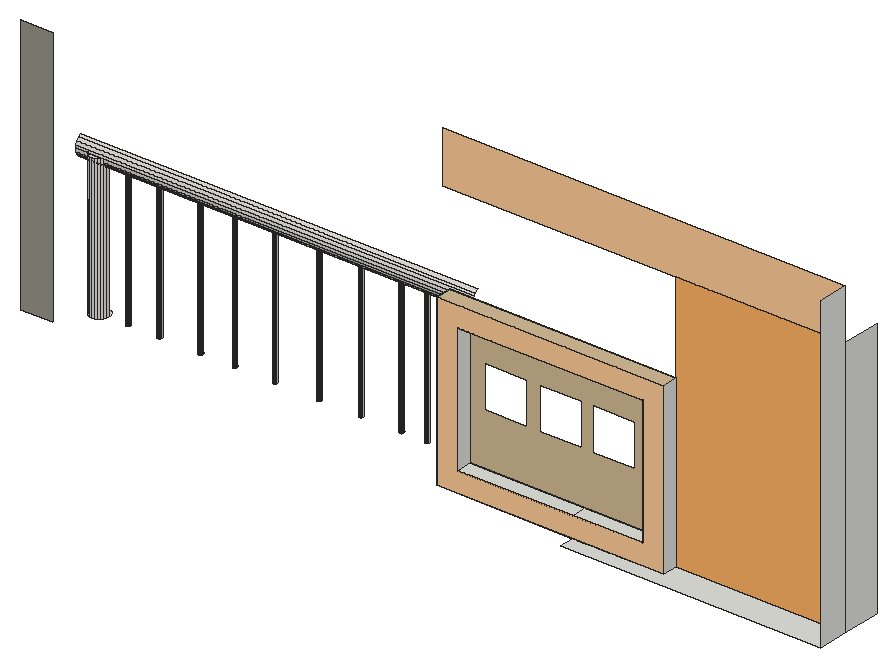
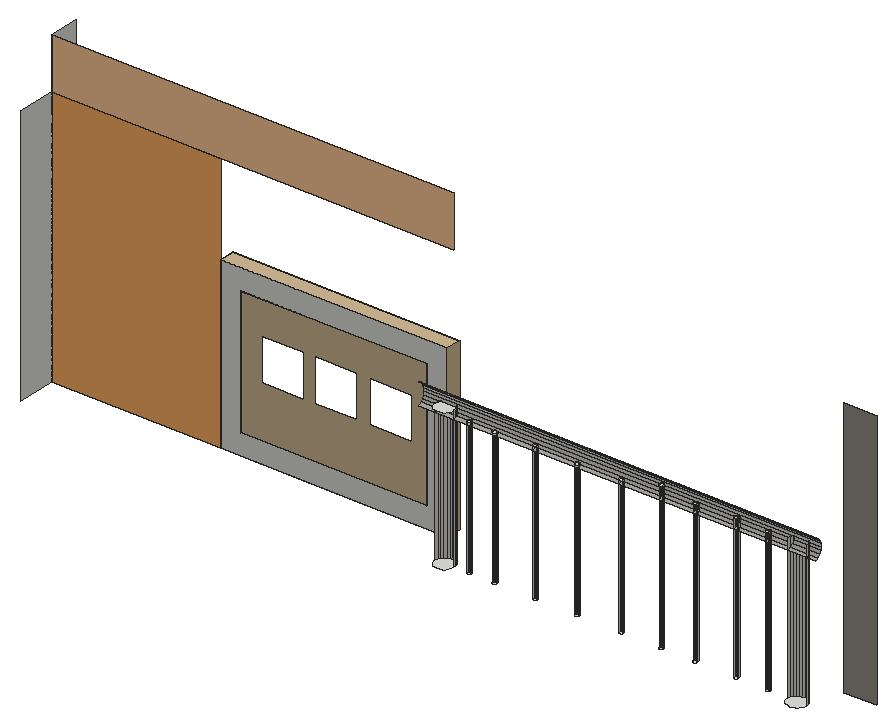
# SketchUp Ruby script. Lengths in inches.
U = 1.inch
M = Sketchup.active_model
def pt(a) = Geom::Point3d.new(a.map { |v| v * U })
def face(e, loops, mat)
  f = e.add_face(loops[0].map { |a| pt(a) })
  loops[1..].each { |l| e.add_face(l.map { |a| pt(a) }).erase! }
  f.material = f.back_material = mat if mat
  f
end
# faces: each face lists its corners as indices into pts; further lists are holes
def faces(e, pts, list, mat = nil) = list.each { |f| face(e, (f[0].is_a?(Array) ? f : [f]).map { |l| l.map { |i| pts[i] } }, mat) }
# xy, xz, yz: faces in a plane at the given z, y or x. An outline is a flat list of corners, or four numbers for a rectangle; further outlines are holes
def ring(l) = l.size == 4 ? [[l[0], l[1]], [l[2], l[1]], [l[2], l[3]], [l[0], l[3]]] : l.each_slice(2).to_a
def flat(e, list, mat, &to3) = list.each { |f| face(e, (f[0].is_a?(Array) ? f : [f]).map { |l| ring(l).map { |u, v| to3.(u, v) } }, mat) }
def xy(e, z, list, mat = nil) = flat(e, list, mat) { |x, y| [x, y, z] }
def xz(e, y, list, mat = nil) = flat(e, list, mat) { |x, z| [x, y, z] }
def yz(e, x, list, mat = nil) = flat(e, list, mat) { |y, z| [x, y, z] }
def lines(e, pts, list) = list.each { |a, b| e.add_line(pt(pts[a]), pt(pts[b])) }
# prism: a flat outline (further loops are holes) pulled along v
def prism(e, loops, v, mat = nil)
  f = face(e, loops, mat); d = Geom::Vector3d.new(v.map { |x| x * U })
  f.pushpull(f.normal.samedirection?(d) ? d.length : -d.length)
end
def box(e, o, s, mat = nil) = prism(e, [[o, [o[0] + s[0], o[1], o[2]], [o[0] + s[0], o[1] + s[1], o[2]], [o[0], o[1] + s[1], o[2]]]], [0, 0, s[2]], mat)
def at(x, y, z, deg = 0) = Geom::Transformation.translation(pt([x, y, z])) * Geom::Transformation.rotation(ORIGIN, Z_AXIS, deg.degrees)
def axes(o, x, y, z) = Geom::Transformation.new([*x, 0, *y, 0, *z, 0, *pt(o).to_a, 1])
def part(name) = M.definitions.add(name)
# library, detail: a bought-in or finely detailed component or shape, given as its bounding box
def library(name, o, s) = part(name).tap { |d| box(d.entities, o, s) }
def detail(e, o, s) = box(e.add_group.entities, o, s)
def put(e, d, t, mat = nil) = e.add_instance(d, t).tap { |i| i.material = mat if mat }
def group(e, t, mat = nil) = e.add_group.tap { |g| g.transformation = t; g.material = mat if mat }.entities
root = M.entities
M.materials.add("[Color C02]").color = [255, 204, 153]
M.materials.add("[Color C03]").color = [255, 178, 101]
M.materials.add("[Formica Beige]").color = [211, 187, 149]
M.materials.add("[Formica Graystone]").color = [149, 146, 135]
M.materials.add("[Terrazzo Tile Light]").color = [219, 217, 210]
xy(root,120,[[156.76,33.14,228.875,33.14,228.875,41.58,181.98,41.58,181.98,37.33,156.76,37.33],[119.1,37.33,156.76,41.58],[156.76,37.33,181.98,41.58],[14.33,48.46,13.65,48.55,13.02,48.81,12.48,49.23,12.06,49.77,11.8,50.4,11.71,51.08,11.8,51.76,12.06,52.4,12.48,52.9375,13.02,53.36,13.65,53.62,14.33,53.71,15.01,53.62,15.64,53.36,16.1875,52.9375,16.6,52.4,16.87,51.76,16.96,51.08,16.87,50.4,16.6,49.77,16.1875,49.23,15.64,48.81,15.01,48.55],[112.21,48.46,111.53,48.55,110.89,48.81,110.35,49.23,109.93,49.77,109.67,50.4,109.58,51.08,109.67,51.76,109.93,52.4,110.35,52.9375,110.89,53.36,111.53,53.62,112.21,53.71,112.89,53.62,113.52,53.36,114.0625,52.9375,114.48,52.4,114.74,51.76,114.83,51.08,114.74,50.4,114.48,49.77,114.0625,49.23,113.52,48.81,112.89,48.55],
  [22.54,50.32,22.4,50.34,22.26,50.4,22.14,50.48,22.05,50.6,22,50.74,21.98,50.88,22,51.03,22.05,51.16,22.14,51.28,22.26,51.37,22.4,51.43,22.54,51.44,22.6875,51.43,22.82,51.37,22.94,51.28,23.03,51.16,23.09,51.03,23.1,50.88,23.09,50.74,23.03,50.6,22.94,50.48,22.82,50.4,22.6875,50.34],[31.29,50.32,31.15,50.34,31.01,50.4,30.89,50.48,30.8,50.6,30.75,50.74,30.73,50.88,30.75,51.03,30.8,51.16,30.89,51.28,31.01,51.37,31.15,51.43,31.29,51.44,31.4375,51.43,31.57,51.37,31.69,51.28,31.78,51.16,31.84,51.03,31.85,50.88,31.84,50.74,31.78,50.6,31.69,50.48,31.57,50.4,31.4375,50.34],[42.67,50.32,42.52,50.34,42.39,50.4,42.27,50.48,42.18,50.6,42.125,50.74,42.1,50.88,42.125,51.03,42.18,51.16,42.27,51.28,42.39,51.37,42.52,51.43,42.67,51.44,42.8125,51.43,42.95,51.37,43.06,51.28,43.15,51.16,43.21,51.03,43.23,50.88,43.21,50.74,43.15,50.6,43.06,50.48,42.95,50.4,42.8125,50.34],[52.1,50.32,51.96,50.34,51.82,50.4,51.71,50.48,51.62,50.6,51.5625,50.74,51.54,50.88,51.5625,51.03,51.62,51.16,51.71,51.28,51.82,51.37,51.96,51.43,52.1,51.44,52.25,51.43,52.39,51.37,52.5,51.28,52.59,51.16,52.65,51.03,52.67,50.88,52.65,50.74,52.59,50.6,52.5,50.48,52.39,50.4,52.25,50.34],[63.23,50.32,63.08,50.34,62.95,50.4,62.83,50.48,62.74,50.6,62.6875,50.74,62.67,50.88,62.6875,51.03,62.74,51.16,62.83,51.28,62.95,51.37,63.08,51.43,63.23,51.44,63.375,51.43,63.51,51.37,63.63,51.28,63.72,51.16,63.77,51.03,63.79,50.88,63.77,50.74,63.72,50.6,63.63,50.48,63.51,50.4,63.375,50.34],
  [75.6,50.32,75.46,50.34,75.32,50.4,75.21,50.48,75.12,50.6,75.0625,50.74,75.04,50.88,75.0625,51.03,75.12,51.16,75.21,51.28,75.32,51.37,75.46,51.43,75.6,51.44,75.75,51.43,75.89,51.37,76,51.28,76.09,51.16,76.15,51.03,76.17,50.88,76.15,50.74,76.09,50.6,76,50.48,75.89,50.4,75.75,50.34],[87.1,50.32,86.96,50.34,86.82,50.4,86.71,50.48,86.62,50.6,86.5625,50.74,86.54,50.88,86.5625,51.03,86.62,51.16,86.71,51.28,86.82,51.37,86.96,51.43,87.1,51.44,87.25,51.43,87.39,51.37,87.5,51.28,87.59,51.16,87.65,51.03,87.67,50.88,87.65,50.74,87.59,50.6,87.5,50.48,87.39,50.4,87.25,50.34],[98.42,50.32,98.27,50.34,98.14,50.4,98.02,50.48,97.93,50.6,97.875,50.74,97.85,50.88,97.875,51.03,97.93,51.16,98.02,51.28,98.14,51.37,98.27,51.43,98.42,51.44,98.5625,51.43,98.7,51.37,98.81,51.28,98.9,51.16,98.96,51.03,98.98,50.88,98.96,50.74,98.9,50.6,98.81,50.48,98.7,50.4,98.5625,50.34],[105.42,50.32,105.27,50.34,105.14,50.4,105.02,50.48,104.93,50.6,104.875,50.74,104.85,50.88,104.875,51.03,104.93,51.16,105.02,51.28,105.14,51.37,105.27,51.43,105.42,51.44,105.5625,51.43,105.7,51.37,105.81,51.28,105.9,51.16,105.96,51.03,105.98,50.88,105.96,50.74,105.9,50.6,105.81,50.48,105.7,50.4,105.5625,50.34]])
xy(root,125.72,[[124.82,37.33,156.76,41.58],[156.76,37.33,176.26,41.58]])
xy(root,157.5625,[[98.42,50.32,98.5625,50.34,98.7,50.4,98.81,50.48,98.9,50.6,98.96,50.74,98.98,50.88,98.96,51.03,98.9,51.16,98.81,51.28,98.7,51.37,98.5625,51.43,98.42,51.44,98.27,51.43,98.14,51.37,98.02,51.28,97.93,51.16,97.875,51.03,97.85,50.88,97.875,50.74,97.93,50.6,98.02,50.48,98.14,50.4,98.27,50.34]])
xy(root,157.625,[[75.6,50.32,75.75,50.34,75.89,50.4,76,50.48,76.09,50.6,76.15,50.74,76.17,50.88,76.15,51.03,76.09,51.16,76,51.28,75.89,51.37,75.75,51.43,75.6,51.44,75.46,51.43,75.32,51.37,75.21,51.28,75.12,51.16,75.0625,51.03,75.04,50.88,75.0625,50.74,75.12,50.6,75.21,50.48,75.32,50.4,75.46,50.34]])
xy(root,157.8125,[[105.42,50.32,105.5625,50.34,105.7,50.4,105.81,50.48,105.9,50.6,105.96,50.74,105.98,50.88,105.96,51.03,105.9,51.16,105.81,51.28,105.7,51.37,105.5625,51.43,105.42,51.44,105.27,51.43,105.14,51.37,105.02,51.28,104.93,51.16,104.875,51.03,104.85,50.88,104.875,50.74,104.93,50.6,105.02,50.48,105.14,50.4,105.27,50.34]])
xy(root,158.09,[[63.23,50.32,63.375,50.34,63.51,50.4,63.63,50.48,63.72,50.6,63.77,50.74,63.79,50.88,63.77,51.03,63.72,51.16,63.63,51.28,63.51,51.37,63.375,51.43,63.23,51.44,63.08,51.43,62.95,51.37,62.83,51.28,62.74,51.16,62.6875,51.03,62.67,50.88,62.6875,50.74,62.74,50.6,62.83,50.48,62.95,50.4,63.08,50.34]])
xy(root,158.1875,[[87.1,50.32,87.25,50.34,87.39,50.4,87.5,50.48,87.59,50.6,87.65,50.74,87.67,50.88,87.65,51.03,87.59,51.16,87.5,51.28,87.39,51.37,87.25,51.43,87.1,51.44,86.96,51.43,86.82,51.37,86.71,51.28,86.62,51.16,86.5625,51.03,86.54,50.88,86.5625,50.74,86.62,50.6,86.71,50.48,86.82,50.4,86.96,50.34]])
xy(root,159,[[112.21,48.46,112.89,48.55,113.52,48.81,114.0625,49.23,114.48,49.77,114.74,50.4,114.83,51.08,114.74,51.76,114.48,52.4,114.0625,52.9375,113.52,53.36,112.89,53.62,112.21,53.71,111.53,53.62,110.89,53.36,110.35,52.9375,109.93,52.4,109.67,51.76,109.58,51.08,109.67,50.4,109.93,49.77,110.35,49.23,110.89,48.81,111.53,48.55]])
xy(root,159.4375,[[42.67,50.32,42.8125,50.34,42.95,50.4,43.06,50.48,43.15,50.6,43.21,50.74,43.23,50.88,43.21,51.03,43.15,51.16,43.06,51.28,42.95,51.37,42.8125,51.43,42.67,51.44,42.52,51.43,42.39,51.37,42.27,51.28,42.18,51.16,42.125,51.03,42.1,50.88,42.125,50.74,42.18,50.6,42.27,50.48,42.39,50.4,42.52,50.34]])
xy(root,159.5,[[22.54,50.32,22.6875,50.34,22.82,50.4,22.94,50.48,23.03,50.6,23.09,50.74,23.1,50.88,23.09,51.03,23.03,51.16,22.94,51.28,22.82,51.37,22.6875,51.43,22.54,51.44,22.4,51.43,22.26,51.37,22.14,51.28,22.05,51.16,22,51.03,21.98,50.88,22,50.74,22.05,50.6,22.14,50.48,22.26,50.4,22.4,50.34]])
xy(root,159.78,[[14.33,48.46,15.01,48.55,15.64,48.81,16.1875,49.23,16.42,49.53,12.24,49.53,12.48,49.23,13.02,48.81,13.65,48.55]])
xy(root,159.875,[[31.29,50.32,31.4375,50.34,31.57,50.4,31.69,50.48,31.78,50.6,31.84,50.74,31.85,50.88,31.84,51.03,31.78,51.16,31.69,51.28,31.57,51.37,31.4375,51.43,31.29,51.44,31.15,51.43,31.01,51.37,30.89,51.28,30.8,51.16,30.75,51.03,30.73,50.88,30.75,50.74,30.8,50.6,30.89,50.48,31.01,50.4,31.15,50.34]])
xy(root,160.66,[[52.1,50.32,52.25,50.34,52.39,50.4,52.5,50.48,52.59,50.6,52.65,50.74,52.67,50.88,52.65,51.03,52.59,51.16,52.5,51.28,52.39,51.37,52.25,51.43,52.1,51.44,51.96,51.43,51.82,51.37,51.71,51.28,51.62,51.16,51.5625,51.03,51.54,50.88,51.5625,50.74,51.62,50.6,51.71,50.48,51.82,50.4,51.96,50.34]])
xy(root,161.21,[[124.82,37.33,176.26,41.58]])
xy(root,166.92,[[119.1,37.33,181.98,41.58]],"[Formica Beige]")
xz(root,37.33,[[[119.1,120,181.98,166.92],[124.82,125.72,176.26,161.21]]],"[Color C02]")
xz(root,41.58,[[[119.1,120,181.98,166.92],[124.82,125.72,176.26,161.21]]])
xz(root,41.58,[[117.3125,192,228.875,206.25]],"[Color C02]")
xz(root,41.58,[[181.98,120,228.875,192]],"[Color C03]")
xz(root,41.58,[[[124.82,125.72,176.26,161.21],[128.8125,140.26,140.5625,152.01],[158.8125,140.26,170.5625,152.01],[144.125,140.26,155.875,152.01]]],"[Formica Beige]")
xz(root,41.58,[[0,120,9,192]],"[Formica Graystone]")
yz(root,119.1,[[37.33,120,41.58,166.92]],"[Formica Beige]")
yz(root,124.82,[[37.33,125.72,41.58,161.21]])
yz(root,176.26,[[37.33,125.72,41.58,161.21]])
yz(root,181.98,[[37.33,120,41.58,166.92]])
yz(root,228.875,[[33.14,120,41.58,206.25],[41.58,120,52.39,192]])
p = [[13.02,48.81,120],[13.65,48.55,120],[13.65,48.55,159.78],[13.02,48.81,159.78],[14.33,48.46,120],[14.33,48.46,159.78],
  [15.01,48.55,120],[15.01,48.55,159.78],[15.64,48.81,120],[15.64,48.81,159.78],[110.89,48.81,120],[111.53,48.55,120],
  [111.53,48.55,159],[110.89,48.81,159],[112.21,48.46,120],[112.21,48.46,159],[112.89,48.55,120],[112.89,48.55,159],
  [113.52,48.81,120],[113.52,48.81,159],[12.48,49.23,120],[12.48,49.23,159.78],[16.1875,49.23,120],[16.1875,49.23,159.78],
  [110.35,49.23,120],[110.35,49.23,159],[114.0625,49.23,120],[114.0625,49.23,159],[12.06,49.77,120],[12.24,49.53,159.78],
  [12.06,49.77,159.78],[16.6,49.77,120],[16.6,49.77,159.78],[16.42,49.53,159.78],[109.93,49.77,120],[109.93,49.77,159],
  [114.48,49.77,120],[114.48,49.77,159],[11.8,50.4,120],[11.8,50.4,159.78],[16.87,50.4,120],[16.87,50.4,159.78],
  [109.67,50.4,120],[109.67,50.4,159],[114.74,50.4,120],[114.74,50.4,159],[22.26,50.4,120],[22.4,50.34,120],
  [22.4,50.34,159.5],[22.26,50.4,159.5],[22.54,50.32,120],[22.54,50.32,159.5],[22.6875,50.34,120],[22.6875,50.34,159.5],
  [22.82,50.4,120],[22.82,50.4,159.5],[31.01,50.4,120],[31.15,50.34,120],[31.15,50.34,159.875],[31.01,50.4,159.875],
  [31.29,50.32,120],[31.29,50.32,159.875],[31.4375,50.34,120],[31.4375,50.34,159.875],[31.57,50.4,120],[31.57,50.4,159.875],
  [42.39,50.4,120],[42.52,50.34,120],[42.52,50.34,159.4375],[42.39,50.4,159.4375],[42.67,50.32,120],[42.67,50.32,159.4375],
  [42.8125,50.34,120],[42.8125,50.34,159.4375],[42.95,50.4,120],[42.95,50.4,159.4375],[51.82,50.4,120],[51.96,50.34,120],
  [51.96,50.34,160.66],[51.82,50.4,160.66],[52.1,50.32,120],[52.1,50.32,160.66],[52.25,50.34,120],[52.25,50.34,160.66],
  [52.39,50.4,120],[52.39,50.4,160.66],[62.95,50.4,120],[63.08,50.34,120],[63.08,50.34,158.09],[62.95,50.4,158.09],
  [63.23,50.32,120],[63.23,50.32,158.09],[63.375,50.34,120],[63.375,50.34,158.09],[63.51,50.4,120],[63.51,50.4,158.09],
  [75.32,50.4,120],[75.46,50.34,120],[75.46,50.34,157.625],[75.32,50.4,157.625],[75.6,50.32,120],[75.6,50.32,157.625],
  [75.75,50.34,120],[75.75,50.34,157.625],[75.89,50.4,120],[75.89,50.4,157.625],[86.82,50.4,120],[86.96,50.34,120],
  [86.96,50.34,158.1875],[86.82,50.4,158.1875],[87.1,50.32,120],[87.1,50.32,158.1875],[87.25,50.34,120],[87.25,50.34,158.1875],
  [87.39,50.4,120],[87.39,50.4,158.1875],[98.14,50.4,120],[98.27,50.34,120],[98.27,50.34,157.5625],[98.14,50.4,157.5625],
  [98.42,50.32,120],[98.42,50.32,157.5625],[98.5625,50.34,120],[98.5625,50.34,157.5625],[98.7,50.4,120],[98.7,50.4,157.5625],
  [105.14,50.4,120],[105.27,50.34,120],[105.27,50.34,157.8125],[105.14,50.4,157.8125],[105.42,50.32,120],[105.42,50.32,157.8125],
  [105.5625,50.34,120],[105.5625,50.34,157.8125],[105.7,50.4,120],[105.7,50.4,157.8125],[11.71,51.08,120],[11.71,51.08,159.78],
  [16.96,51.08,120],[16.96,51.08,159.78],[22.14,50.48,120],[22.14,50.48,159.5],[22.94,50.48,120],[22.94,50.48,159.5],
  [30.89,50.48,120],[30.89,50.48,159.875],[31.69,50.48,120],[31.69,50.48,159.875],[42.27,50.48,120],[42.27,50.48,159.4375],
  [43.06,50.48,120],[43.06,50.48,159.4375],[51.71,50.48,120],[51.71,50.48,160.66],[52.5,50.48,120],[52.5,50.48,160.66],
  [62.83,50.48,120],[62.83,50.48,158.09],[63.63,50.48,120],[63.63,50.48,158.09],[75.21,50.48,120],[75.21,50.48,157.625],
  [76,50.48,120],[76,50.48,157.625],[86.71,50.48,120],[86.71,50.48,158.1875],[87.5,50.48,120],[87.5,50.48,158.1875],
  [98.02,50.48,120],[98.02,50.48,157.5625],[98.81,50.48,120],[98.81,50.48,157.5625],[105.02,50.48,120],[105.02,50.48,157.8125],
  [105.81,50.48,120],[105.81,50.48,157.8125],[109.58,51.08,120],[109.58,51.08,159],[114.83,51.08,120],[114.83,51.08,159],
  [22.05,50.6,120],[22.05,50.6,159.5],[23.03,50.6,120],[23.03,50.6,159.5],[30.8,50.6,120],[30.8,50.6,159.875],
  [31.78,50.6,120],[31.78,50.6,159.875],[42.18,50.6,120],[42.18,50.6,159.4375],[43.15,50.6,120],[43.15,50.6,159.4375],
  [51.62,50.6,120],[51.62,50.6,160.66],[52.59,50.6,120],[52.59,50.6,160.66],[62.74,50.6,120],[62.74,50.6,158.09],
  [63.72,50.6,120],[63.72,50.6,158.09],[75.12,50.6,120],[75.12,50.6,157.625],[76.09,50.6,120],[76.09,50.6,157.625],
  [86.62,50.6,120],[86.62,50.6,158.1875],[87.59,50.6,120],[87.59,50.6,158.1875],[97.93,50.6,120],[97.93,50.6,157.5625],
  [98.9,50.6,120],[98.9,50.6,157.5625],[104.93,50.6,120],[104.93,50.6,157.8125],[105.9,50.6,120],[105.9,50.6,157.8125],
  [22,50.74,120],[22,50.74,159.5],[23.09,50.74,120],[23.09,50.74,159.5],[30.75,50.74,120],[30.75,50.74,159.875],
  [31.84,50.74,120],[31.84,50.74,159.875],[42.125,50.74,120],[42.125,50.74,159.4375],[43.21,50.74,120],[43.21,50.74,159.4375],
  [51.5625,50.74,120],[51.5625,50.74,160.66],[52.65,50.74,120],[52.65,50.74,160.66],[62.6875,50.74,120],[62.6875,50.74,158.09],
  [63.77,50.74,120],[63.77,50.74,158.09],[75.0625,50.74,120],[75.0625,50.74,157.625],[76.15,50.74,120],[76.15,50.74,157.625],
  [86.5625,50.74,120],[86.5625,50.74,158.1875],[87.65,50.74,120],[87.65,50.74,158.1875],[97.875,50.74,120],[97.875,50.74,157.5625],
  [98.96,50.74,120],[98.96,50.74,157.5625],[104.875,50.74,120],[104.875,50.74,157.8125],[105.96,50.74,120],[105.96,50.74,157.8125],
  [21.98,50.88,120],[21.98,50.88,159.5],[23.1,50.88,120],[23.1,50.88,159.5],[30.73,50.88,120],[30.73,50.88,159.875],
  [31.85,50.88,120],[31.85,50.88,159.875],[42.1,50.88,120],[42.1,50.88,159.4375],[43.23,50.88,120],[43.23,50.88,159.4375],
  [51.54,50.88,120],[51.54,50.88,160.66],[52.67,50.88,120],[52.67,50.88,160.66],[62.67,50.88,120],[62.67,50.88,158.09],
  [63.79,50.88,120],[63.79,50.88,158.09],[75.04,50.88,120],[75.04,50.88,157.625],[76.17,50.88,120],[76.17,50.88,157.625],
  [86.54,50.88,120],[86.54,50.88,158.1875],[87.67,50.88,120],[87.67,50.88,158.1875],[97.85,50.88,120],[97.85,50.88,157.5625],
  [98.98,50.88,120],[98.98,50.88,157.5625],[104.85,50.88,120],[104.85,50.88,157.8125],[105.98,50.88,120],[105.98,50.88,157.8125],
  [22,51.03,120],[22,51.03,159.5],[23.09,51.03,120],[23.09,51.03,159.5],[30.75,51.03,120],[30.75,51.03,159.875],
  [31.84,51.03,120],[31.84,51.03,159.875],[42.125,51.03,120],[42.125,51.03,159.4375],[43.21,51.03,120],[43.21,51.03,159.4375],
  [51.5625,51.03,120],[51.5625,51.03,160.66],[52.65,51.03,120],[52.65,51.03,160.66],[62.6875,51.03,120],[62.6875,51.03,158.09],
  [63.77,51.03,120],[63.77,51.03,158.09],[75.0625,51.03,120],[75.0625,51.03,157.625],[76.15,51.03,120],[76.15,51.03,157.625],
  [86.5625,51.03,120],[86.5625,51.03,158.1875],[87.65,51.03,120],[87.65,51.03,158.1875],[97.875,51.03,120],[97.875,51.03,157.5625],
  [98.96,51.03,120],[98.96,51.03,157.5625],[104.875,51.03,120],[104.875,51.03,157.8125],[105.96,51.03,120],[105.96,51.03,157.8125],
  [22.05,51.16,120],[22.05,51.16,159.5],[23.03,51.16,120],[23.03,51.16,159.5],[30.8,51.16,120],[30.8,51.16,159.875],
  [31.78,51.16,120],[31.78,51.16,159.875],[119.1,51.22,156.86],[119.1,50.52,157.4],[9,50.52,157.4],[9,51.22,156.86],
  [119.1,49.98,158.09],[9,49.98,158.09],[119.1,49.64,158.91],[9,49.64,158.91],[119.1,49.53,159.78],[9,49.53,159.78],
  [119.1,49.64,160.66],[9,49.64,160.66],[119.1,49.98,161.47],[9,49.98,161.47],[119.1,50.52,162.17],[9,50.52,162.17],
  [119.1,51.22,162.7],[9,51.22,162.7]]
faces(root,p,[[0,1,2,3],[1,4,5,2],[4,6,7,5],[6,8,9,7],[10,11,12,13],[11,14,15,12],[14,16,17,15],[16,18,19,17],
  [20,0,3,21],[8,22,23,9],[24,10,13,25],[18,26,27,19],[28,20,21,29,30],[22,31,32,33,23],[34,24,25,35],[26,36,37,27],
  [38,28,30,39],[31,40,41,32],[42,34,35,43],[36,44,45,37],[46,47,48,49],[47,50,51,48],[50,52,53,51],[52,54,55,53],
  [56,57,58,59],[57,60,61,58],[60,62,63,61],[62,64,65,63],[66,67,68,69],[67,70,71,68],[70,72,73,71],[72,74,75,73],
  [76,77,78,79],[77,80,81,78],[80,82,83,81],[82,84,85,83],[86,87,88,89],[87,90,91,88],[90,92,93,91],[92,94,95,93],
  [96,97,98,99],[97,100,101,98],[100,102,103,101],[102,104,105,103],[106,107,108,109],[107,110,111,108],[110,112,113,111],[112,114,115,113],
  [116,117,118,119],[117,120,121,118],[120,122,123,121],[122,124,125,123],[126,127,128,129],[127,130,131,128],[130,132,133,131],[132,134,135,133],
  [136,38,39,137],[40,138,139,41],[140,46,49,141],[54,142,143,55],[144,56,59,145],[64,146,147,65],[148,66,69,149],[74,150,151,75],
  [152,76,79,153],[84,154,155,85],[156,86,89,157],[94,158,159,95],[160,96,99,161],[104,162,163,105],[164,106,109,165],[114,166,167,115],
  [168,116,119,169],[124,170,171,125],[172,126,129,173],[134,174,175,135],[176,42,43,177],[44,178,179,45],[180,140,141,181],[142,182,183,143],
  [184,144,145,185],[146,186,187,147],[188,148,149,189],[150,190,191,151],[192,152,153,193],[154,194,195,155],[196,156,157,197],[158,198,199,159],
  [200,160,161,201],[162,202,203,163],[204,164,165,205],[166,206,207,167],[208,168,169,209],[170,210,211,171],[212,172,173,213],[174,214,215,175],
  [216,180,181,217],[182,218,219,183],[220,184,185,221],[186,222,223,187],[224,188,189,225],[190,226,227,191],[228,192,193,229],[194,230,231,195],
  [232,196,197,233],[198,234,235,199],[236,200,201,237],[202,238,239,203],[240,204,205,241],[206,242,243,207],[244,208,209,245],[210,246,247,211],
  [248,212,213,249],[214,250,251,215],[252,216,217,253],[218,254,255,219],[256,220,221,257],[222,258,259,223],[260,224,225,261],[226,262,263,227],
  [264,228,229,265],[230,266,267,231],[268,232,233,269],[234,270,271,235],[272,236,237,273],[238,274,275,239],[276,240,241,277],[242,278,279,243],
  [280,244,245,281],[246,282,283,247],[284,248,249,285],[250,286,287,251],[288,252,253,289],[254,290,291,255],[292,256,257,293],[258,294,295,259],
  [296,260,261,297],[262,298,299,263],[300,264,265,301],[266,302,303,267],[304,268,269,305],[270,306,307,271],[308,272,273,309],[274,310,311,275],
  [312,276,277,313],[278,314,315,279],[316,280,281,317],[282,318,319,283],[320,284,285,321],[286,322,323,287],[324,288,289,325],[290,326,327,291],
  [328,292,293,329],[294,330,331,295],[332,333,334,335],[333,336,337,334],[336,338,339,337],[338,340,33,29,341,339],[340,342,343,341,29,33],[342,344,345,343],
  [344,346,347,345],[346,348,349,347]],"[Terrazzo Tile Light]")
